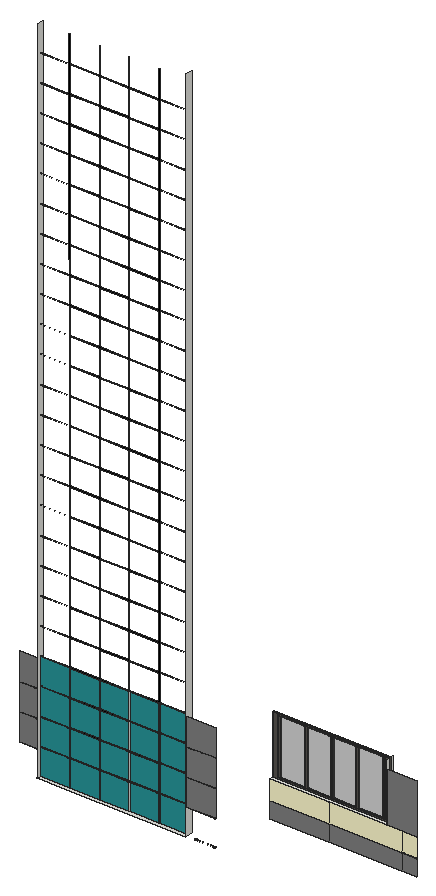
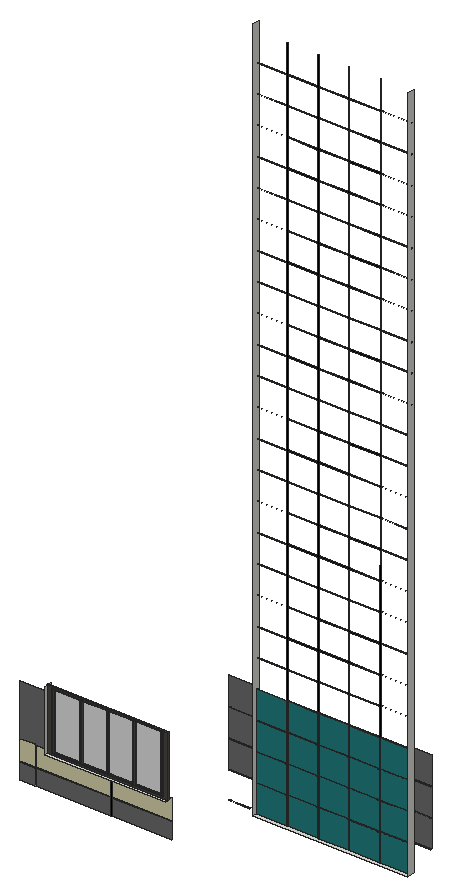
# SketchUp Ruby script. Lengths in inches.
U = 1.inch
M = Sketchup.active_model
def pt(a) = Geom::Point3d.new(a.map { |v| v * U })
def face(e, loops, mat)
  f = e.add_face(loops[0].map { |a| pt(a) })
  loops[1..].each { |l| e.add_face(l.map { |a| pt(a) }).erase! }
  f.material = f.back_material = mat if mat
  f
end
# faces: each face lists its corners as indices into pts; further lists are holes
def faces(e, pts, list, mat = nil) = list.each { |f| face(e, (f[0].is_a?(Array) ? f : [f]).map { |l| l.map { |i| pts[i] } }, mat) }
# xy, xz, yz: faces in a plane at the given z, y or x. An outline is a flat list of corners, or four numbers for a rectangle; further outlines are holes
def ring(l) = l.size == 4 ? [[l[0], l[1]], [l[2], l[1]], [l[2], l[3]], [l[0], l[3]]] : l.each_slice(2).to_a
def flat(e, list, mat, &to3) = list.each { |f| face(e, (f[0].is_a?(Array) ? f : [f]).map { |l| ring(l).map { |u, v| to3.(u, v) } }, mat) }
def xy(e, z, list, mat = nil) = flat(e, list, mat) { |x, y| [x, y, z] }
def xz(e, y, list, mat = nil) = flat(e, list, mat) { |x, z| [x, y, z] }
def yz(e, x, list, mat = nil) = flat(e, list, mat) { |y, z| [x, y, z] }
def lines(e, pts, list) = list.each { |a, b| e.add_line(pt(pts[a]), pt(pts[b])) }
# prism: a flat outline (further loops are holes) pulled along v
def prism(e, loops, v, mat = nil)
  f = face(e, loops, mat); d = Geom::Vector3d.new(v.map { |x| x * U })
  f.pushpull(f.normal.samedirection?(d) ? d.length : -d.length)
end
def box(e, o, s, mat = nil) = prism(e, [[o, [o[0] + s[0], o[1], o[2]], [o[0] + s[0], o[1] + s[1], o[2]], [o[0], o[1] + s[1], o[2]]]], [0, 0, s[2]], mat)
def at(x, y, z, deg = 0) = Geom::Transformation.translation(pt([x, y, z])) * Geom::Transformation.rotation(ORIGIN, Z_AXIS, deg.degrees)
def axes(o, x, y, z) = Geom::Transformation.new([*x, 0, *y, 0, *z, 0, *pt(o).to_a, 1])
def part(name) = M.definitions.add(name)
# library, detail: a bought-in or finely detailed component or shape, given as its bounding box
def library(name, o, s) = part(name).tap { |d| box(d.entities, o, s) }
def detail(e, o, s) = box(e.add_group.entities, o, s)
def put(e, d, t, mat = nil) = e.add_instance(d, t).tap { |i| i.material = mat if mat }
def group(e, t, mat = nil) = e.add_group.tap { |g| g.transformation = t; g.material = mat if mat }.entities
root = M.entities
M.materials.add("Aluminum_Anodized_DarkGray").color = [87, 83, 78]
M.materials.add("Glass_Coated_Black").color = [65, 65, 65]
M.materials["Glass_Coated_Black"].alpha = 0.42
M.materials.add("[0050_LemonChiffon]").color = [255, 250, 205]
M.materials.add("[0081_CadetBlue]").color = [40, 149, 153]
M.materials.add("[0133_Gray]").color = [128, 128, 128]
M.materials.add("[0137_Black]").color = [0, 0, 0]
c1 = part("Group\#2")
xy(c1.entities,0,[[0,0,54,3]],"Aluminum_Anodized_DarkGray")
xy(c1.entities,2,[[2.25,0,51.75,1],[2.25,2,51.75,3]],"Aluminum_Anodized_DarkGray")
xy(c1.entities,3,[[3.375,1,14.625,1.5],[15.75,1,26.4375,1.5],[27.5625,1,38.25,1.5],[39.375,1,50.625,1.5],[3.375,1.5,14.625,2],
  [15.75,1.5,26.4375,2],[27.5625,1.5,38.25,2],[39.375,1.5,50.625,2]],"Aluminum_Anodized_DarkGray")
xy(c1.entities,99,[[3.375,1,14.625,1.5],[15.75,1,26.4375,1.5],[26.4375,1,27.5625,2],[27.5625,1,38.25,1.5],[38.25,1,39.375,2],
  [39.375,1,50.625,1.5],[3.375,1.5,14.625,2],[15.75,1.5,26.4375,2],[27.5625,1.5,38.25,2],[39.375,1.5,50.625,2]],"Aluminum_Anodized_DarkGray")
xy(c1.entities,100,[[2.25,0,51.75,1],[2.25,2,51.75,3]],"Aluminum_Anodized_DarkGray")
xy(c1.entities,102,[[0,0,54,3]],"Aluminum_Anodized_DarkGray")
xz(c1.entities,0,[[[0,0,54,102],[2.25,2,51.75,100]]],"Aluminum_Anodized_DarkGray")
xz(c1.entities,1,[[[2.25,2,51.75,100],[39.375,3,50.625,99],[3.375,3,14.625,99],[27.5625,3,38.25,99],[15.75,3,26.4375,99]]],"Aluminum_Anodized_DarkGray")
xz(c1.entities,1.5,[[3.375,3,14.625,99],[15.75,3,27,99],[27.5625,3,38.8125,99],[39.375,3,50.625,99]],"Glass_Coated_Black")
xz(c1.entities,2,[[[2.25,2,51.75,100],[39.375,3,50.625,99],[3.375,3,14.625,99],[27.5625,3,38.25,99],[15.75,3,26.4375,99]]],"Aluminum_Anodized_DarkGray")
xz(c1.entities,3,[[[0,0,54,102],[2.25,2,51.75,100]]],"Aluminum_Anodized_DarkGray")
yz(c1.entities,0,[[0,0,3,102]],"Aluminum_Anodized_DarkGray")
yz(c1.entities,2.25,[[0,2,1,100],[2,2,3,100]],"Aluminum_Anodized_DarkGray")
yz(c1.entities,3.375,[[1,3,1.5,99],[1.5,3,2,99]],"Aluminum_Anodized_DarkGray")
yz(c1.entities,14.625,[[1,3,1.5,99],[1.5,3,2,99]],"Aluminum_Anodized_DarkGray")
yz(c1.entities,15.75,[[1,3,1.5,99],[1.5,3,2,99]],"Aluminum_Anodized_DarkGray")
yz(c1.entities,26.4375,[[1,3,2,99]],"Aluminum_Anodized_DarkGray")
yz(c1.entities,27.5625,[[1,3,1.5,99],[1.5,3,2,99]],"Aluminum_Anodized_DarkGray")
yz(c1.entities,38.25,[[1,3,2,99]],"Aluminum_Anodized_DarkGray")
yz(c1.entities,39.375,[[1,3,1.5,99],[1.5,3,2,99]],"Aluminum_Anodized_DarkGray")
yz(c1.entities,50.625,[[1,3,1.5,99],[1.5,3,2,99]],"Aluminum_Anodized_DarkGray")
yz(c1.entities,51.75,[[0,2,1,100],[2,2,3,100]],"Aluminum_Anodized_DarkGray")
yz(c1.entities,54,[[0,0,3,102]],"Aluminum_Anodized_DarkGray")
p = [[15.75,2,99],[14.625,2,99]]
lines(c1.entities,p,[[0,1]])
xy(root,165,[[136.75,221.1875,136.9375,221.6875],[[137.25,221.1875,137.25,221.6875,136.9375,221.6875,136.9375,230.1875,319.9375,230.1875,319.9375,221.1875,161.25,221.1875,161.25,221.6875,160.75,221.6875,160.75,221.1875],[210.01,225.49,210.51,225.6875],[246.05,225.49,246.55,225.6875],[283.09,225.49,283.59,225.6875],[173.04,225.49,173.48,225.6875]],[173.04,225.49,173.48,225.6875],[210.01,225.49,210.51,225.6875],[246.05,225.49,246.55,225.6875],
  [283.09,225.49,283.59,225.6875]])
xy(root,165.25,[[330.6875,221.1875,355.9375,221.6875]])
xy(root,165.75,[[330.1875,221.1875,355.9375,221.6875]])
xy(root,197.24,[[115.9375,221.1875,136.9375,221.6875],[319.9375,221.1875,355.9375,221.6875]])
xy(root,197.74,[[115.9375,221.1875,136.9375,221.6875],[136.9,225.49,173.04,225.6875],[173.4375,225.49,210.01,225.6875],[210.51,225.49,246.05,225.6875],[246.55,225.49,283.09,225.6875],
  [283.59,225.49,319.625,225.6875]])
xy(root,197.74,[[319.9375,221.1875,355.9375,221.6875]],"[0137_Black]")
xy(root,198.24,[[136.9,225.49,173.04,225.6875],[173.4375,225.49,210.01,225.6875],[210.51,225.49,246.05,225.6875],[246.55,225.49,283.09,225.6875],[283.59,225.49,319.625,225.6875]])
xy(root,204,[[355.9375,305.1875,499.37,314.1875]])
xy(root,230.48,[[115.9375,221.1875,136.9375,221.6875],[319.9375,221.1875,355.9375,221.6875]])
xy(root,230.98,[[115.9375,221.1875,136.9375,221.6875],[319.9375,221.1875,355.9375,221.6875],[136.86,225.49,173.04,225.6875],[173.4,225.49,210.01,225.6875],[210.51,225.49,246.05,225.6875],
  [246.55,225.49,283.09,225.6875],[283.59,225.49,319.625,225.6875]])
xy(root,231.48,[[136.86,225.49,173.04,225.6875],[173.4,225.49,210.01,225.6875],[210.51,225.49,246.05,225.6875],[246.55,225.49,283.09,225.6875],[283.59,225.49,319.625,225.6875]])
xy(root,263.72,[[115.9375,221.1875,136.9375,221.6875],[319.9375,221.1875,355.9375,221.6875]])
xy(root,264.22,[[115.9375,221.1875,136.9375,221.6875],[319.9375,221.1875,355.9375,221.6875],[136.83,225.49,173.04,225.6875],[173.36,225.49,210.01,225.6875],[210.51,225.49,246.05,225.6875],
  [246.55,225.49,283.09,225.6875],[283.59,225.49,319.625,225.6875]])
xy(root,264.72,[[136.83,225.49,173.04,225.6875],[173.36,225.49,210.01,225.6875],[210.51,225.49,246.05,225.6875],[246.55,225.49,283.09,225.6875],[283.59,225.49,319.625,225.6875]])
xz(root,221.1875,[[115.9375,197.74,136.9375,230.48],[319.9375,197.74,355.9375,230.48],[115.9375,230.98,136.9375,263.72],[319.9375,230.98,355.9375,263.72],[115.9375,264.22,136.9375,297.46],
  [319.9375,264.22,355.9375,297.46]],"[0133_Gray]")
xz(root,221.6875,[[115.9375,197.24,136.9375,197.74],[115.9375,230.48,136.9375,230.98],[115.9375,263.72,136.9375,264.22]])
xz(root,221.6875,[[319.9375,197.24,355.9375,197.74],[319.9375,230.48,355.9375,230.98],[319.9375,263.72,355.9375,264.22]],"[0137_Black]")
xz(root,225.49,[[[173.04,165,173.48,165,173.4375,197.74,210.01,197.74,210.01,165,210.51,165,210.51,197.74,246.05,197.74,246.05,165,246.55,165,246.55,197.74,283.09,197.74,283.09,165,283.59,165,283.59,197.74,319.625,197.74,319.625,198.24,283.59,198.24,283.59,230.98,319.625,230.98,319.625,231.48,283.59,231.48,283.59,264.22,319.625,264.22,319.625,264.72,283.59,264.72,283.59,297.46,319.625,297.46,319.625,297.96,283.59,297.96,283.59,330.7,319.625,330.7,319.625,331.2,283.59,331.2,283.59,363.94,319.625,363.94,319.625,364.44,283.59,364.44,283.59,397.18,319.625,397.18,319.625,397.68,283.59,397.68,283.59,430.42,319.625,430.42,319.625,430.92,283.59,430.92,283.59,463.66,319.625,463.66,319.625,464.16,283.59,464.16,283.59,496.9,319.625,496.9,319.625,497.4,283.59,497.4,283.59,530.14,319.625,530.14,319.625,530.64,283.59,530.64,283.59,563.38,319.625,563.38,319.625,563.88,283.59,563.88,283.59,596.62,319.625,596.62,319.625,597.12,283.59,597.12,283.59,629.86,319.625,629.86,319.625,630.36,283.59,630.36,283.59,663.1,319.625,663.1,319.625,663.6,283.59,663.6,283.59,696.34,319.625,696.34,319.625,696.84,283.59,696.84,283.59,729.58,319.625,729.58,319.625,730.08,283.59,730.08,283.59,762.82,319.625,762.82,319.625,763.32,283.59,763.32,283.59,796.06,319.625,796.06,319.625,796.56,283.59,796.56,283.59,829.3,319.625,829.3,319.625,829.8,283.59,829.8,283.59,862.54,319.625,862.54,319.625,863.04,283.59,863.04,283.59,895.78,319.625,895.78,319.625,896.28,283.59,896.28,283.59,929.02,319.625,929.02,319.625,929.52,283.59,929.52,283.59,962.26,319.625,962.26,319.625,962.76,283.59,962.76,283.59,996,283.09,996,283.09,962.76,246.55,962.76,246.55,996,246.05,996,246.05,962.76,210.51,962.76,210.51,996,210.01,996,210.01,962.76,173.04,962.76,173.04,996,172.54,996,172.58,962.76,136.04,962.76,136.04,962.26,172.58,962.26,172.61,929.52,136.08,929.52,136.08,929.02,172.61,929.02,172.65,896.28,136.11,896.28,136.11,895.78,172.65,895.78,172.6875,863.04,136.15,863.04,136.15,862.54,172.6875,862.54,172.73,829.8,136.1875,829.8,136.1875,829.3,172.73,829.3,172.76,796.56,136.23,796.56,136.23,796.06,172.76,796.06,172.8,763.32,136.26,763.32,136.26,762.82,172.8,762.82,172.84,730.08,136.3,730.08,136.3,729.58,172.84,729.58,172.875,696.84,136.34,696.84,136.34,696.34,172.875,696.34,172.91,663.6,136.375,663.6,136.375,663.1,172.91,663.1,172.95,630.36,136.41,630.36,136.41,629.86,172.95,629.86,172.99,597.12,136.45,597.12,136.45,596.62,172.99,596.62,173.02,563.88,136.49,563.88,136.49,563.38,173.03,563.38,173.04,552.8,173.04,563.38,210.01,563.38,210.01,530.64,173.0625,530.64,173.04,552.8,173.04,530.64,136.52,530.64,136.52,530.14,173.04,530.14,173.04,497.4,136.5625,497.4,136.5625,496.9,173.04,496.9,173.04,464.16,136.6,464.16,136.6,463.66,173.04,463.66,173.04,430.92,136.64,430.92,136.64,430.42,173.04,430.42,173.04,397.68,136.67,397.68,136.68,397.18,173.04,397.18,173.04,364.44,136.71,364.44,136.71,363.94,173.04,363.94,173.04,331.2,136.75,331.2,136.75,330.7,173.04,330.7,173.04,297.96,136.79,297.96,136.79,297.46,173.04,297.46,173.04,264.72,136.83,264.72,136.83,264.22,173.04,264.22,173.04,231.48,136.86,231.48,136.86,230.98,173.04,230.98,173.04,198.24,136.9,198.24,136.9,197.74,173.04,197.74],[173.04,896.28,210.01,929.02],[173.04,563.88,210.01,596.62],[173.04,663.6,210.01,696.34],[173.04,929.52,210.01,962.26],[173.04,796.56,210.01,829.3],[173.04,863.04,210.01,895.78],[173.04,696.84,210.01,729.58],[173.04,763.32,210.01,796.06],[173.04,829.8,210.01,862.54],[173.04,630.36,210.01,663.1],[173.04,597.12,210.01,629.86],[173.04,730.08,210.01,762.82],[173.1,497.4,173.0625,530.14,210.01,530.14,210.01,497.4],[173.14,464.16,173.1,496.9,210.01,496.9,210.01,464.16],[173.18,430.92,173.14,463.66,210.01,463.66,210.01,430.92],[173.21,397.68,173.18,430.42,210.01,430.42,210.01,397.68],[173.25,364.44,173.21,397.18,210.01,397.18,210.01,364.44],[173.29,331.2,173.25,363.94,210.01,363.94,210.01,331.2],[173.33,297.96,173.29,330.7,210.01,330.7,210.01,297.96],[173.36,264.72,173.33,297.46,210.01,297.46,210.01,264.72],[173.4,231.48,173.36,264.22,210.01,264.22,210.01,231.48],[173.4375,198.24,173.4,230.98,210.01,230.98,210.01,198.24],[246.55,896.28,283.09,929.02],[246.55,663.6,283.09,696.34],[246.55,929.52,283.09,962.26],[246.55,796.56,283.09,829.3],[246.55,563.88,283.09,596.62],[246.55,464.16,283.09,496.9],[246.55,297.96,283.09,330.7],[246.55,264.72,283.09,297.46],[246.55,231.48,283.09,264.22],[246.55,397.68,283.09,430.42],[246.55,198.24,283.09,230.98],[246.55,364.44,283.09,397.18],[246.55,530.64,283.09,563.38],[246.55,497.4,283.09,530.14],[246.55,430.92,283.09,463.66],[246.55,331.2,283.09,363.94],[246.55,630.36,283.09,663.1],[246.55,829.8,283.09,862.54],[246.55,863.04,283.09,895.78],[246.55,763.32,283.09,796.06],[246.55,696.84,283.09,729.58],[246.55,597.12,283.09,629.86],[246.55,730.08,283.09,762.82],[210.51,896.28,246.05,929.02],[210.51,663.6,246.05,696.34],[210.51,929.52,246.05,962.26],[210.51,796.56,246.05,829.3],[210.51,563.88,246.05,596.62],[210.51,464.16,246.05,496.9],[210.51,264.72,246.05,297.46],[210.51,231.48,246.05,264.22],[210.51,297.96,246.05,330.7],[210.51,198.24,246.05,230.98],[210.51,364.44,246.05,397.18],[210.51,397.68,246.05,430.42],[210.51,530.64,246.05,563.38],[210.51,497.4,246.05,530.14],[210.51,430.92,246.05,463.66],[210.51,331.2,246.05,363.94],[210.51,597.12,246.05,629.86],[210.51,630.36,246.05,663.1],[210.51,763.32,246.05,796.06],[210.51,829.8,246.05,862.54],[210.51,863.04,246.05,895.78],[210.51,696.84,246.05,729.58],[210.51,730.08,246.05,762.82]]],"[0137_Black]")
xz(root,225.6875,[[136.9375,165,173.04,165,173.04,197.74,136.9,197.74],[173.48,165,210.01,165,210.01,197.74,173.4375,197.74],[210.51,165,246.05,197.74],[246.55,165,283.09,197.74],[283.59,165,319.625,197.74],
  [136.9,198.24,173.04,198.24,173.04,230.98,136.86,230.98],[173.4375,198.24,210.01,198.24,210.01,230.98,173.4,230.98],[210.51,198.24,246.05,230.98],[246.55,198.24,283.09,230.98],[283.59,198.24,319.625,230.98],
  [136.86,231.48,173.04,231.48,173.04,264.22,136.83,264.22],[173.4,231.48,210.01,231.48,210.01,264.22,173.36,264.22],[210.51,231.48,246.05,264.22],[246.55,231.48,283.09,264.22],[283.59,231.48,319.625,264.22],
  [136.83,264.72,173.04,264.72,173.04,297.46,136.79,297.46],[173.36,264.72,210.01,264.72,210.01,297.46,173.33,297.46],[210.51,264.72,246.05,297.46],[246.55,264.72,283.09,297.46],[283.59,264.72,319.625,297.46]],"[0081_CadetBlue]")
xz(root,305.1875,[[517.9375,160,518.4375,179.5],[517.9375,179.5,518.4375,180],[518.4375,179.5,535.9375,180],[517.9375,180,518.4375,204]])
xz(root,305.1875,[[355.9375,180,427.65,204],[428.15,180,517.9375,204],[518.4375,180,535.9375,204]],"[0050_LemonChiffon]")
xz(root,305.1875,[[355.9375,160,427.65,179.5],[428.15,160,517.9375,179.5],[518.4375,160,535.9375,179.5],[499.37,204,535.9375,265.64]],"[0133_Gray]")
xz(root,305.1875,[[427.65,160,428.15,160,428.15,179.5,517.9375,179.5,517.9375,180,428.15,180,428.15,204,427.65,204,427.65,180,355.9375,180,355.9375,179.5,427.65,179.5]],"[0137_Black]")
yz(root,136.83,[[225.49,264.22,225.6875,264.72]])
yz(root,136.86,[[225.49,230.98,225.6875,231.48]])
yz(root,136.9,[[225.49,197.74,225.6875,198.24]])
yz(root,136.9375,[[221.1875,165,230.1875,165,230.1875,996,221.1875,996,221.1875,962.26,221.6875,962.26,221.6875,961.76,221.1875,961.76,221.1875,929.02,221.6875,929.02,221.6875,928.52,221.1875,928.52,221.1875,895.78,221.6875,895.78,221.6875,895.28,221.1875,895.28,221.1875,862.54,221.6875,862.54,221.6875,862.04,221.1875,862.04,221.1875,829.3,221.6875,829.3,221.6875,828.8,221.1875,828.8,221.1875,796.56,221.6875,796.56,221.6875,796.04,221.1875,796.04,221.1875,763.32,221.6875,763.32,221.6875,762.82,221.1875,762.82,221.1875,729.58,221.6875,729.58,221.6875,729.08,221.1875,729.08,221.1875,696.84,221.6875,696.84,221.6875,696.34,221.1875,696.34,221.1875,663.6,221.6875,663.6,221.6875,663.1,221.1875,663.1,221.1875,629.86,221.6875,629.86,221.6875,629.36,221.1875,629.36,221.1875,596.62,221.6875,596.62,221.6875,596.12,221.1875,596.12,221.1875,563.38,221.6875,563.38,221.6875,562.88,221.1875,562.88,221.1875,530.64,221.6875,530.64,221.6875,530.14,221.1875,530.14,221.1875,496.9,221.6875,496.9,221.6875,496.4,221.1875,496.4,221.1875,463.66,221.6875,463.66,221.6875,463.16,221.1875,463.16,221.1875,430.88,221.6875,430.88,221.6875,430.42,221.1875,430.42,221.1875,397.68,221.6875,397.68,221.6875,397.18,221.1875,397.18,221.1875,364.44,221.6875,364.44,221.6875,363.94,221.1875,363.94,221.1875,330.7,221.6875,330.7,221.6875,330.2,221.1875,330.2,221.1875,297.96,221.6875,297.96,221.6875,297.46,221.1875,297.46,221.1875,264.22,221.6875,264.22,221.6875,263.72,221.1875,263.72,221.1875,230.98,221.6875,230.98,221.6875,230.48,221.1875,230.48,221.1875,197.74,221.6875,197.74,221.6875,197.24,221.1875,197.24]])
yz(root,173.04,[[225.49,165,225.6875,197.74],[225.49,198.24,225.6875,230.98],[225.49,231.48,225.6875,264.22],[225.49,264.72,225.6875,297.46]])
yz(root,210.01,[[225.49,165,225.6875,197.74],[225.49,198.24,225.6875,230.98],[225.49,231.48,225.6875,264.22],[225.49,264.72,225.6875,297.46]])
yz(root,210.51,[[225.49,165,225.6875,197.74],[225.49,198.24,225.6875,230.98],[225.49,231.48,225.6875,264.22],[225.49,264.72,225.6875,297.46]])
yz(root,246.05,[[225.49,165,225.6875,197.74],[225.49,198.24,225.6875,230.98],[225.49,231.48,225.6875,264.22],[225.49,264.72,225.6875,297.46]])
yz(root,246.55,[[225.49,165,225.6875,197.74],[225.49,198.24,225.6875,230.98],[225.49,231.48,225.6875,264.22],[225.49,264.72,225.6875,297.46]])
yz(root,283.09,[[225.49,165,225.6875,197.74],[225.49,198.24,225.6875,230.98],[225.49,231.48,225.6875,264.22],[225.49,264.72,225.6875,297.46]])
yz(root,283.59,[[225.49,165,225.6875,197.74],[225.49,198.24,225.6875,230.98],[225.49,231.48,225.6875,264.22],[225.49,264.72,225.6875,297.46]])
yz(root,319.625,[[225.49,197.74,225.6875,198.24],[225.49,230.98,225.6875,231.48],[225.49,264.22,225.6875,264.72]])
yz(root,319.9375,[[221.1875,165,221.1875,197.24,221.6875,197.24,221.6875,197.74,221.1875,197.74,221.1875,230.48,221.6875,230.48,221.6875,230.98,221.1875,230.98,221.1875,263.72,221.6875,263.72,221.6875,264.22,221.1875,264.22,221.1875,297.46,221.6875,297.46,221.6875,297.96,221.1875,297.96,221.1875,330.2,221.6875,330.2,221.6875,330.7,221.1875,330.7,221.1875,363.94,221.6875,363.94,221.6875,364.44,221.1875,364.44,221.1875,397.18,221.6875,397.18,221.6875,397.68,221.1875,397.68,221.1875,430.42,221.3125,430.42,221.3125,430.92,221.1875,430.92,221.1875,463.16,221.3125,463.16,221.3125,463.66,221.1875,463.66,221.1875,496.4,221.25,496.4,221.25,496.9,221.1875,496.9,221.1875,530.14,221.75,530.14,221.75,530.64,221.1875,530.64,221.1875,562.88,221.6875,562.88,221.6875,563.38,221.1875,563.38,221.1875,596.12,221.6875,596.12,221.6875,596.62,221.1875,596.62,221.1875,629.36,221.6875,629.36,221.6875,629.86,221.1875,629.86,221.1875,663.1,221.6875,663.1,221.6875,663.6,221.1875,663.6,221.1875,696.34,221.6875,696.34,221.6875,696.84,221.1875,696.84,221.1875,729.08,221.6875,729.08,221.6875,729.58,221.1875,729.58,221.1875,762.82,221.6875,762.82,221.6875,763.32,221.1875,763.32,221.1875,796.06,221.6875,796.06,221.6875,796.56,221.1875,796.56,221.1875,828.8,221.6875,828.8,221.6875,829.3,221.1875,829.3,221.1875,862.04,221.6875,862.04,221.6875,862.54,221.1875,862.54,221.1875,895.28,221.6875,895.28,221.6875,895.78,221.1875,895.78,221.1875,928.52,221.6875,928.52,221.6875,929.02,221.1875,929.02,221.1875,961.76,221.6875,961.76,221.6875,962.26,221.1875,962.26,221.1875,1005,230.1875,1005,230.1875,165]])
yz(root,499.37,[[305.1875,204,314.1875,276.01]])
p = [[173.48,225.6875,165],[173.4375,225.6875,197.74],[173.4375,225.49,197.74],[173.48,225.49,165],[173.4375,225.6875,198.24],[173.4,225.6875,230.98],
  [173.4,225.49,230.98],[173.4375,225.49,198.24],[173.4,225.6875,231.48],[173.36,225.6875,264.22],[173.36,225.49,264.22],[173.4,225.49,231.48],
  [173.36,225.6875,264.72],[173.33,225.6875,297.46],[173.33,225.49,297.46],[173.36,225.49,264.72]]
faces(root,p,[[0,1,2,3],[4,5,6,7],[8,9,10,11],[12,13,14,15]])
put(root,c1,axes([355.9375,309.6875,204],[2.66667,0,0],[0,0.5,0],[0,0,0.71]))
